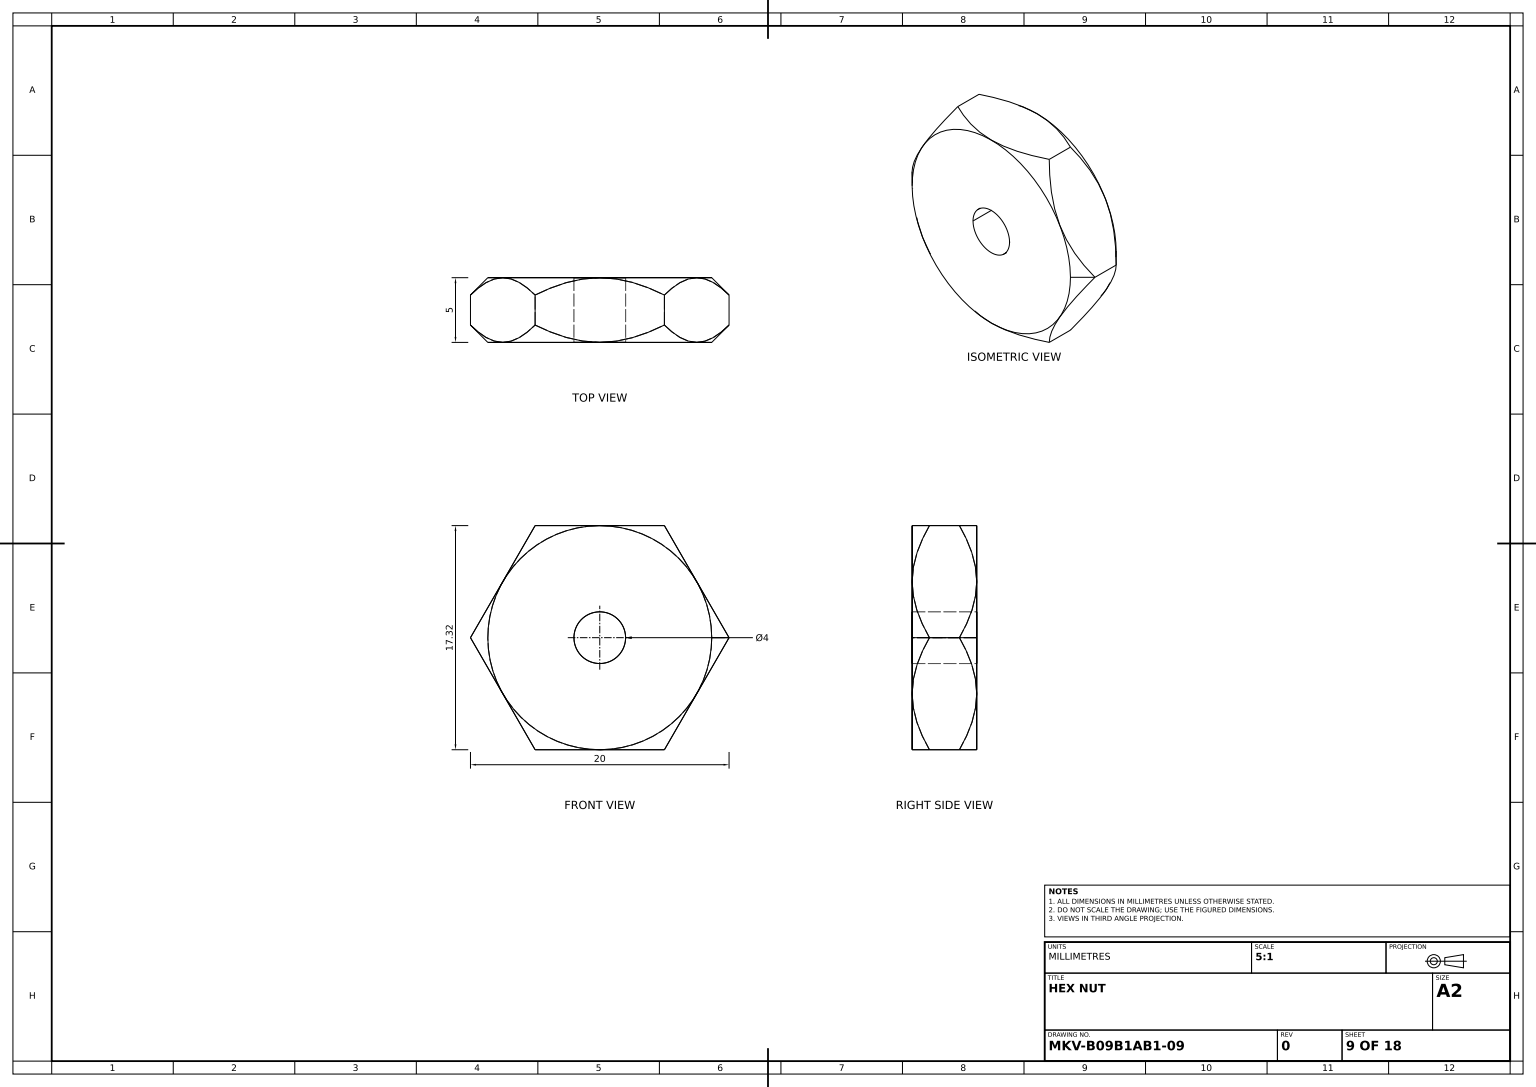
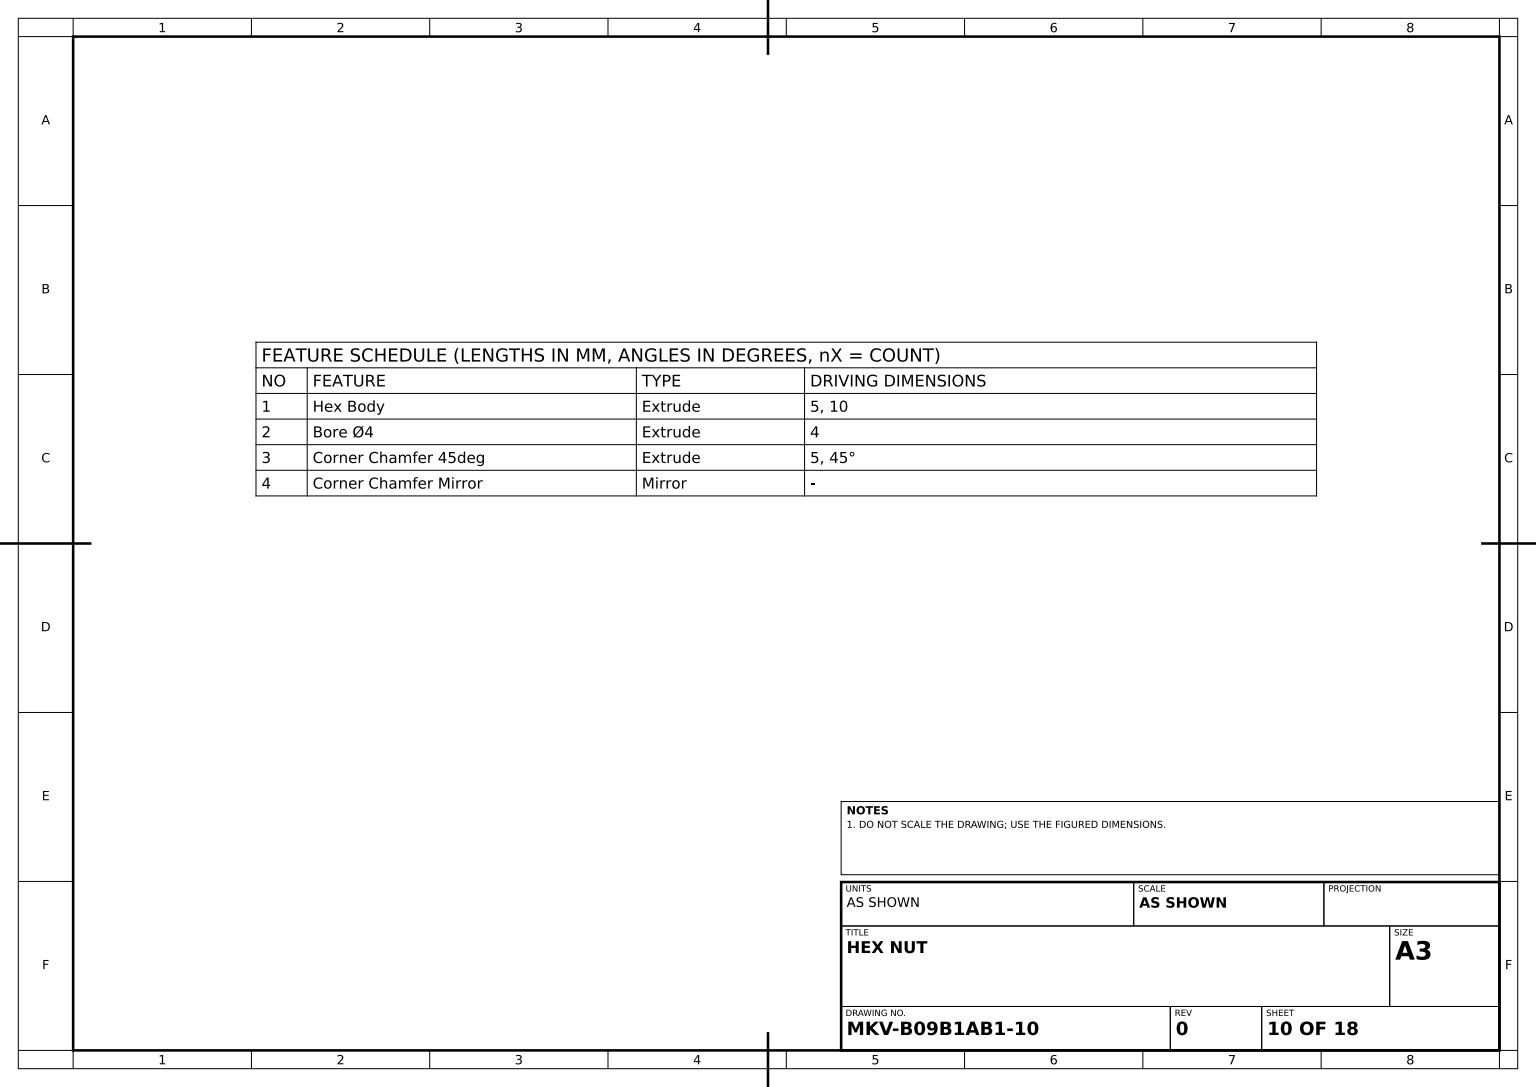
ISO-10303-21;
HEADER;
FILE_DESCRIPTION((''),'2;1');
FILE_NAME('','',(''),(''),'','','');
FILE_SCHEMA(('AUTOMOTIVE_DESIGN'));
ENDSEC;
DATA;
#1=APPLICATION_CONTEXT('');
#2=PRODUCT_CONTEXT('',#1,'mechanical');
#3=PRODUCT('','','',(#2));
#4=PRODUCT_DEFINITION_FORMATION('','',#3);
#5=PRODUCT_DEFINITION_CONTEXT('',#1,'design');
#6=PRODUCT_DEFINITION('','',#4,#5);
#7=PRODUCT_DEFINITION_SHAPE('','',#6);
#8=(LENGTH_UNIT()NAMED_UNIT(*)SI_UNIT(.MILLI.,.METRE.));
#9=(NAMED_UNIT(*)PLANE_ANGLE_UNIT()SI_UNIT($,.RADIAN.));
#10=(NAMED_UNIT(*)SI_UNIT($,.STERADIAN.)SOLID_ANGLE_UNIT());
#11=UNCERTAINTY_MEASURE_WITH_UNIT(LENGTH_MEASURE(1.E-05),#8,'distance_accuracy_value','');
#12=(GEOMETRIC_REPRESENTATION_CONTEXT(3)GLOBAL_UNCERTAINTY_ASSIGNED_CONTEXT((#11))GLOBAL_UNIT_ASSIGNED_CONTEXT((#8,#9,#10))REPRESENTATION_CONTEXT('',''));
#13=CARTESIAN_POINT('',(-5.,8.660254,1.160254));
#14=VERTEX_POINT('',#13);
#15=CARTESIAN_POINT('',(-5.,8.660254,-1.160254));
#16=VERTEX_POINT('',#15);
#17=CARTESIAN_POINT('',(-5.,8.660254,2.5));
#18=DIRECTION('',(0.,0.,-1.));
#19=VECTOR('',#18,1000.);
#20=LINE('',#17,#19);
#21=EDGE_CURVE('',#14,#16,#20,.T.);
#22=ORIENTED_EDGE('',*,*,#21,.F.);
#23=CARTESIAN_POINT('',(0.,8.660254,2.5));
#24=VERTEX_POINT('',#23);
#25=CARTESIAN_POINT('',(-0.873275,8.660254,2.5));
#26=CARTESIAN_POINT('',(-1.729188,8.660254,2.366037));
#27=CARTESIAN_POINT('',(-2.992496,8.660254,2.006453));
#28=CARTESIAN_POINT('',(-3.408399,8.660254,1.860772));
#29=CARTESIAN_POINT('',(-4.216688,8.660254,1.535097));
#30=CARTESIAN_POINT('',(-4.611749,8.660254,1.354379));
#31=B_SPLINE_CURVE_WITH_KNOTS('',3,(#23,#25,#26,#27,#28,#29,#30,#13),.UNSPECIFIED.,.F.,.F.,(4,2,2,4),(0.019209283,0.021821739,0.023127967,0.024434195),.UNSPECIFIED.);
#32=EDGE_CURVE('',#24,#14,#31,.T.);
#33=ORIENTED_EDGE('',*,*,#32,.F.);
#34=CARTESIAN_POINT('',(5.,8.660254,1.160254));
#35=VERTEX_POINT('',#34);
#36=CARTESIAN_POINT('',(4.223723,8.660254,1.548393));
#37=CARTESIAN_POINT('',(3.409694,8.660254,1.887275));
#38=CARTESIAN_POINT('',(2.159803,8.660254,2.243681));
#39=CARTESIAN_POINT('',(1.737019,8.660254,2.337768));
#40=CARTESIAN_POINT('',(0.876568,8.660254,2.466153));
#41=CARTESIAN_POINT('',(0.435084,8.660254,2.5));
#42=B_SPLINE_CURVE_WITH_KNOTS('',3,(#34,#36,#37,#38,#39,#40,#41,#23),.UNSPECIFIED.,.F.,.F.,(4,2,2,4),(0.01400296,0.016606121,0.017907702,0.019209283),.UNSPECIFIED.);
#43=EDGE_CURVE('',#35,#24,#42,.T.);
#44=ORIENTED_EDGE('',*,*,#43,.F.);
#45=CARTESIAN_POINT('',(5.,8.660254,-1.160254));
#46=VERTEX_POINT('',#45);
#47=CARTESIAN_POINT('',(5.,8.660254,2.5));
#48=LINE('',#47,#19);
#49=EDGE_CURVE('',#35,#46,#48,.T.);
#50=ORIENTED_EDGE('',*,*,#49,.T.);
#51=CARTESIAN_POINT('',(0.,8.660254,-2.5));
#52=VERTEX_POINT('',#51);
#53=CARTESIAN_POINT('',(4.223723,8.660254,-1.548393));
#54=CARTESIAN_POINT('',(3.409694,8.660254,-1.887275));
#55=CARTESIAN_POINT('',(2.159803,8.660254,-2.243681));
#56=CARTESIAN_POINT('',(1.737019,8.660254,-2.337768));
#57=CARTESIAN_POINT('',(0.876568,8.660254,-2.466153));
#58=CARTESIAN_POINT('',(0.435084,8.660254,-2.5));
#59=B_SPLINE_CURVE_WITH_KNOTS('',3,(#45,#53,#54,#55,#56,#57,#58,#51),.UNSPECIFIED.,.F.,.F.,(4,2,2,4),(0.01400296,0.016606121,0.017907702,0.019209283),.UNSPECIFIED.);
#60=EDGE_CURVE('',#46,#52,#59,.T.);
#61=ORIENTED_EDGE('',*,*,#60,.T.);
#62=CARTESIAN_POINT('',(-0.873275,8.660254,-2.5));
#63=CARTESIAN_POINT('',(-1.729188,8.660254,-2.366037));
#64=CARTESIAN_POINT('',(-2.992496,8.660254,-2.006453));
#65=CARTESIAN_POINT('',(-3.408399,8.660254,-1.860772));
#66=CARTESIAN_POINT('',(-4.216688,8.660254,-1.535097));
#67=CARTESIAN_POINT('',(-4.611749,8.660254,-1.354379));
#68=B_SPLINE_CURVE_WITH_KNOTS('',3,(#51,#62,#63,#64,#65,#66,#67,#15),.UNSPECIFIED.,.F.,.F.,(4,2,2,4),(0.019209283,0.021821739,0.023127967,0.024434195),.UNSPECIFIED.);
#69=EDGE_CURVE('',#52,#16,#68,.T.);
#70=ORIENTED_EDGE('',*,*,#69,.T.);
#71=EDGE_LOOP('',(#22,#33,#44,#50,#61,#70));
#72=FACE_OUTER_BOUND('',#71,.T.);
#73=DIRECTION('',(0.,-1.,0.));
#74=DIRECTION('',(1.,0.,0.));
#75=AXIS2_PLACEMENT_3D('',#47,#73,#74);
#76=PLANE('',#75);
#77=ADVANCED_FACE('',(#72),#76,.F.);
#78=ORIENTED_EDGE('',*,*,#69,.F.);
#79=CARTESIAN_POINT('',(-7.5,4.330127,-2.5));
#80=VERTEX_POINT('',#79);
#81=CARTESIAN_POINT('',(0.,0.,-2.5));
#82=AXIS2_PLACEMENT_3D('',#81,#18,#74);
#83=CIRCLE('',#82,8.660254);
#84=EDGE_CURVE('',#80,#52,#83,.T.);
#85=ORIENTED_EDGE('',*,*,#84,.F.);
#86=CARTESIAN_POINT('',(-5.392036,7.981228,-1.55229));
#87=CARTESIAN_POINT('',(-5.792944,7.286834,-1.885418));
#88=CARTESIAN_POINT('',(-6.415924,6.207803,-2.241594));
#89=CARTESIAN_POINT('',(-6.627224,5.841819,-2.336146));
#90=CARTESIAN_POINT('',(-7.058806,5.094297,-2.465627));
#91=CARTESIAN_POINT('',(-7.281041,4.709375,-2.5));
#92=B_SPLINE_CURVE_WITH_KNOTS('',3,(#15,#86,#87,#88,#89,#90,#91,#79),.UNSPECIFIED.,.F.,.F.,(4,2,2,4),(0.000000254,0.002591731,0.003887469,0.005183207),.UNSPECIFIED.);
#93=EDGE_CURVE('',#16,#80,#92,.T.);
#94=ORIENTED_EDGE('',*,*,#93,.F.);
#95=EDGE_LOOP('',(#78,#85,#94));
#96=FACE_OUTER_BOUND('',#95,.T.);
#97=DIRECTION('',(0.,0.,1.));
#98=AXIS2_PLACEMENT_3D('',#81,#97,#74);
#99=CONICAL_SURFACE('',#98,8.660254038,0.785398163);
#100=ADVANCED_FACE('',(#96),#99,.T.);
#101=CARTESIAN_POINT('',(-7.5,-4.330127,-2.5));
#102=VERTEX_POINT('',#101);
#103=CARTESIAN_POINT('',(-5.,-8.660254,-1.160254));
#104=VERTEX_POINT('',#103);
#105=CARTESIAN_POINT('',(-7.06515,-5.08331,-2.5));
#106=CARTESIAN_POINT('',(-6.637694,-5.823685,-2.367019));
#107=CARTESIAN_POINT('',(-5.794643,-7.283892,-1.887732));
#108=CARTESIAN_POINT('',(-5.391582,-7.982014,-1.551836));
#109=B_SPLINE_CURVE_WITH_KNOTS('',3,(#101,#105,#106,#107,#108,#103),.UNSPECIFIED.,.F.,.F.,(4,2,4),(0.005183207,0.007756532,0.010329856),.UNSPECIFIED.);
#110=EDGE_CURVE('',#102,#104,#109,.T.);
#111=ORIENTED_EDGE('',*,*,#110,.T.);
#112=CARTESIAN_POINT('',(-5.,-8.660254,1.160254));
#113=VERTEX_POINT('',#112);
#114=CARTESIAN_POINT('',(-5.,-8.660254,2.5));
#115=LINE('',#114,#19);
#116=EDGE_CURVE('',#113,#104,#115,.T.);
#117=ORIENTED_EDGE('',*,*,#116,.F.);
#118=CARTESIAN_POINT('',(-7.5,-4.330127,2.5));
#119=VERTEX_POINT('',#118);
#120=CARTESIAN_POINT('',(-7.06515,-5.08331,2.5));
#121=CARTESIAN_POINT('',(-6.637694,-5.823685,2.367019));
#122=CARTESIAN_POINT('',(-5.794643,-7.283892,1.887732));
#123=CARTESIAN_POINT('',(-5.391582,-7.982014,1.551836));
#124=B_SPLINE_CURVE_WITH_KNOTS('',3,(#118,#120,#121,#122,#123,#112),.UNSPECIFIED.,.F.,.F.,(4,2,4),(0.005183207,0.007756532,0.010329856),.UNSPECIFIED.);
#125=EDGE_CURVE('',#119,#113,#124,.T.);
#126=ORIENTED_EDGE('',*,*,#125,.F.);
#127=CARTESIAN_POINT('',(-10.,0.,1.160254));
#128=VERTEX_POINT('',#127);
#129=CARTESIAN_POINT('',(-9.607964,-0.679026,1.55229));
#130=CARTESIAN_POINT('',(-9.207056,-1.37342,1.885418));
#131=CARTESIAN_POINT('',(-8.584076,-2.452452,2.241594));
#132=CARTESIAN_POINT('',(-8.372776,-2.818435,2.336146));
#133=CARTESIAN_POINT('',(-7.941194,-3.565957,2.465627));
#134=CARTESIAN_POINT('',(-7.718959,-3.950879,2.5));
#135=B_SPLINE_CURVE_WITH_KNOTS('',3,(#127,#129,#130,#131,#132,#133,#134,#118),.UNSPECIFIED.,.F.,.F.,(4,2,2,4),(0.000000254,0.002591731,0.003887469,0.005183207),.UNSPECIFIED.);
#136=EDGE_CURVE('',#128,#119,#135,.T.);
#137=ORIENTED_EDGE('',*,*,#136,.F.);
#138=CARTESIAN_POINT('',(-10.,0.,-1.160254));
#139=VERTEX_POINT('',#138);
#140=CARTESIAN_POINT('',(-10.,0.,2.5));
#141=LINE('',#140,#19);
#142=EDGE_CURVE('',#128,#139,#141,.T.);
#143=ORIENTED_EDGE('',*,*,#142,.T.);
#144=CARTESIAN_POINT('',(-9.607964,-0.679026,-1.55229));
#145=CARTESIAN_POINT('',(-9.207056,-1.37342,-1.885418));
#146=CARTESIAN_POINT('',(-8.584076,-2.452452,-2.241594));
#147=CARTESIAN_POINT('',(-8.372776,-2.818435,-2.336146));
#148=CARTESIAN_POINT('',(-7.941194,-3.565957,-2.465627));
#149=CARTESIAN_POINT('',(-7.718959,-3.950879,-2.5));
#150=B_SPLINE_CURVE_WITH_KNOTS('',3,(#138,#144,#145,#146,#147,#148,#149,#101),.UNSPECIFIED.,.F.,.F.,(4,2,2,4),(0.000000254,0.002591731,0.003887469,0.005183207),.UNSPECIFIED.);
#151=EDGE_CURVE('',#139,#102,#150,.T.);
#152=ORIENTED_EDGE('',*,*,#151,.T.);
#153=EDGE_LOOP('',(#111,#117,#126,#137,#143,#152));
#154=FACE_OUTER_BOUND('',#153,.T.);
#155=DIRECTION('',(0.866025404,0.5,0.));
#156=DIRECTION('',(-0.5,0.866025404,0.));
#157=AXIS2_PLACEMENT_3D('',#140,#155,#156);
#158=PLANE('',#157);
#159=ADVANCED_FACE('',(#154),#158,.F.);
#160=CARTESIAN_POINT('',(-7.5,4.330127,2.5));
#161=VERTEX_POINT('',#160);
#162=CARTESIAN_POINT('',(-7.93485,3.576944,2.5));
#163=CARTESIAN_POINT('',(-8.362306,2.836569,2.367019));
#164=CARTESIAN_POINT('',(-9.205357,1.376362,1.887732));
#165=CARTESIAN_POINT('',(-9.608418,0.67824,1.551836));
#166=B_SPLINE_CURVE_WITH_KNOTS('',3,(#160,#162,#163,#164,#165,#127),.UNSPECIFIED.,.F.,.F.,(4,2,4),(0.005183207,0.007756532,0.010329856),.UNSPECIFIED.);
#167=EDGE_CURVE('',#161,#128,#166,.T.);
#168=ORIENTED_EDGE('',*,*,#167,.T.);
#169=ORIENTED_EDGE('',*,*,#136,.T.);
#170=CARTESIAN_POINT('',(0.,0.,2.5));
#171=AXIS2_PLACEMENT_3D('',#170,#97,#74);
#172=CIRCLE('',#171,8.660254);
#173=EDGE_CURVE('',#161,#119,#172,.T.);
#174=ORIENTED_EDGE('',*,*,#173,.F.);
#175=EDGE_LOOP('',(#168,#169,#174));
#176=FACE_OUTER_BOUND('',#175,.T.);
#177=AXIS2_PLACEMENT_3D('',#170,#18,#74);
#178=CONICAL_SURFACE('',#177,8.660254038,0.785398163);
#179=ADVANCED_FACE('',(#176),#178,.T.);
#180=CARTESIAN_POINT('',(7.5,-4.330127,2.5));
#181=VERTEX_POINT('',#180);
#182=CARTESIAN_POINT('',(10.,0.,1.160254));
#183=VERTEX_POINT('',#182);
#184=CARTESIAN_POINT('',(7.93485,-3.576944,2.5));
#185=CARTESIAN_POINT('',(8.362306,-2.836569,2.367019));
#186=CARTESIAN_POINT('',(9.205357,-1.376362,1.887732));
#187=CARTESIAN_POINT('',(9.608418,-0.67824,1.551836));
#188=B_SPLINE_CURVE_WITH_KNOTS('',3,(#180,#184,#185,#186,#187,#182),.UNSPECIFIED.,.F.,.F.,(4,2,4),(0.005183207,0.007756532,0.010329856),.UNSPECIFIED.);
#189=EDGE_CURVE('',#181,#183,#188,.T.);
#190=ORIENTED_EDGE('',*,*,#189,.T.);
#191=CARTESIAN_POINT('',(8.660254,0.,2.5));
#192=VERTEX_POINT('',#191);
#193=DIRECTION('',(0.707106781,0.,-0.707106781));
#194=VECTOR('',#193,1000.);
#195=LINE('',#191,#194);
#196=EDGE_CURVE('',#192,#183,#195,.T.);
#197=ORIENTED_EDGE('',*,*,#196,.F.);
#198=EDGE_CURVE('',#181,#192,#172,.T.);
#199=ORIENTED_EDGE('',*,*,#198,.F.);
#200=EDGE_LOOP('',(#190,#197,#199));
#201=FACE_OUTER_BOUND('',#200,.T.);
#202=ADVANCED_FACE('',(#201),#178,.T.);
#203=ORIENTED_EDGE('',*,*,#125,.T.);
#204=CARTESIAN_POINT('',(0.,-8.660254,2.5));
#205=VERTEX_POINT('',#204);
#206=CARTESIAN_POINT('',(-4.223723,-8.660254,1.548393));
#207=CARTESIAN_POINT('',(-3.409694,-8.660254,1.887275));
#208=CARTESIAN_POINT('',(-2.159803,-8.660254,2.243681));
#209=CARTESIAN_POINT('',(-1.737019,-8.660254,2.337768));
#210=CARTESIAN_POINT('',(-0.876568,-8.660254,2.466153));
#211=CARTESIAN_POINT('',(-0.435084,-8.660254,2.5));
#212=B_SPLINE_CURVE_WITH_KNOTS('',3,(#112,#206,#207,#208,#209,#210,#211,#204),.UNSPECIFIED.,.F.,.F.,(4,2,2,4),(0.01400296,0.016606121,0.017907702,0.019209283),.UNSPECIFIED.);
#213=EDGE_CURVE('',#113,#205,#212,.T.);
#214=ORIENTED_EDGE('',*,*,#213,.T.);
#215=EDGE_CURVE('',#119,#205,#172,.T.);
#216=ORIENTED_EDGE('',*,*,#215,.F.);
#217=EDGE_LOOP('',(#203,#214,#216));
#218=FACE_OUTER_BOUND('',#217,.T.);
#219=ADVANCED_FACE('',(#218),#178,.T.);
#220=ORIENTED_EDGE('',*,*,#116,.T.);
#221=CARTESIAN_POINT('',(0.,-8.660254,-2.5));
#222=VERTEX_POINT('',#221);
#223=CARTESIAN_POINT('',(-4.223723,-8.660254,-1.548393));
#224=CARTESIAN_POINT('',(-3.409694,-8.660254,-1.887275));
#225=CARTESIAN_POINT('',(-2.159803,-8.660254,-2.243681));
#226=CARTESIAN_POINT('',(-1.737019,-8.660254,-2.337768));
#227=CARTESIAN_POINT('',(-0.876568,-8.660254,-2.466153));
#228=CARTESIAN_POINT('',(-0.435084,-8.660254,-2.5));
#229=B_SPLINE_CURVE_WITH_KNOTS('',3,(#103,#223,#224,#225,#226,#227,#228,#221),.UNSPECIFIED.,.F.,.F.,(4,2,2,4),(0.01400296,0.016606121,0.017907702,0.019209283),.UNSPECIFIED.);
#230=EDGE_CURVE('',#104,#222,#229,.T.);
#231=ORIENTED_EDGE('',*,*,#230,.T.);
#232=CARTESIAN_POINT('',(5.,-8.660254,-1.160254));
#233=VERTEX_POINT('',#232);
#234=CARTESIAN_POINT('',(0.873275,-8.660254,-2.5));
#235=CARTESIAN_POINT('',(1.729188,-8.660254,-2.366037));
#236=CARTESIAN_POINT('',(2.992496,-8.660254,-2.006453));
#237=CARTESIAN_POINT('',(3.408399,-8.660254,-1.860772));
#238=CARTESIAN_POINT('',(4.216688,-8.660254,-1.535097));
#239=CARTESIAN_POINT('',(4.611749,-8.660254,-1.354379));
#240=B_SPLINE_CURVE_WITH_KNOTS('',3,(#221,#234,#235,#236,#237,#238,#239,#232),.UNSPECIFIED.,.F.,.F.,(4,2,2,4),(0.019209283,0.021821739,0.023127967,0.024434195),.UNSPECIFIED.);
#241=EDGE_CURVE('',#222,#233,#240,.T.);
#242=ORIENTED_EDGE('',*,*,#241,.T.);
#243=CARTESIAN_POINT('',(5.,-8.660254,1.160254));
#244=VERTEX_POINT('',#243);
#245=CARTESIAN_POINT('',(5.,-8.660254,2.5));
#246=LINE('',#245,#19);
#247=EDGE_CURVE('',#244,#233,#246,.T.);
#248=ORIENTED_EDGE('',*,*,#247,.F.);
#249=CARTESIAN_POINT('',(0.873275,-8.660254,2.5));
#250=CARTESIAN_POINT('',(1.729188,-8.660254,2.366037));
#251=CARTESIAN_POINT('',(2.992496,-8.660254,2.006453));
#252=CARTESIAN_POINT('',(3.408399,-8.660254,1.860772));
#253=CARTESIAN_POINT('',(4.216688,-8.660254,1.535097));
#254=CARTESIAN_POINT('',(4.611749,-8.660254,1.354379));
#255=B_SPLINE_CURVE_WITH_KNOTS('',3,(#204,#249,#250,#251,#252,#253,#254,#243),.UNSPECIFIED.,.F.,.F.,(4,2,2,4),(0.019209283,0.021821739,0.023127967,0.024434195),.UNSPECIFIED.);
#256=EDGE_CURVE('',#205,#244,#255,.T.);
#257=ORIENTED_EDGE('',*,*,#256,.F.);
#258=ORIENTED_EDGE('',*,*,#213,.F.);
#259=EDGE_LOOP('',(#220,#231,#242,#248,#257,#258));
#260=FACE_OUTER_BOUND('',#259,.T.);
#261=DIRECTION('',(0.,1.,0.));
#262=DIRECTION('',(-1.,0.,0.));
#263=AXIS2_PLACEMENT_3D('',#114,#261,#262);
#264=PLANE('',#263);
#265=ADVANCED_FACE('',(#260),#264,.F.);
#266=CARTESIAN_POINT('',(2.,0.,-2.5));
#267=VERTEX_POINT('',#266);
#268=CARTESIAN_POINT('',(-2.,0.,-2.5));
#269=VERTEX_POINT('',#268);
#270=CIRCLE('',#98,2.);
#271=EDGE_CURVE('',#267,#269,#270,.T.);
#272=ORIENTED_EDGE('',*,*,#271,.F.);
#273=CARTESIAN_POINT('',(2.,0.,2.5));
#274=VERTEX_POINT('',#273);
#275=VECTOR('',#97,1000.);
#276=LINE('',#266,#275);
#277=EDGE_CURVE('',#267,#274,#276,.T.);
#278=ORIENTED_EDGE('',*,*,#277,.T.);
#279=CARTESIAN_POINT('',(-2.,0.,2.5));
#280=VERTEX_POINT('',#279);
#281=CIRCLE('',#171,2.);
#282=EDGE_CURVE('',#274,#280,#281,.T.);
#283=ORIENTED_EDGE('',*,*,#282,.T.);
#284=LINE('',#268,#275);
#285=EDGE_CURVE('',#269,#280,#284,.T.);
#286=ORIENTED_EDGE('',*,*,#285,.F.);
#287=EDGE_LOOP('',(#272,#278,#283,#286));
#288=FACE_OUTER_BOUND('',#287,.T.);
#289=CYLINDRICAL_SURFACE('',#98,2.);
#290=ADVANCED_FACE('',(#288),#289,.F.);
#291=EDGE_CURVE('',#269,#267,#270,.T.);
#292=ORIENTED_EDGE('',*,*,#291,.T.);
#293=ORIENTED_EDGE('',*,*,#271,.T.);
#294=EDGE_LOOP('',(#292,#293));
#295=FACE_BOUND('',#294,.T.);
#296=CARTESIAN_POINT('',(7.5,4.330127,-2.5));
#297=VERTEX_POINT('',#296);
#298=CIRCLE('',#98,8.660254);
#299=EDGE_CURVE('',#297,#52,#298,.T.);
#300=ORIENTED_EDGE('',*,*,#299,.F.);
#301=CARTESIAN_POINT('',(8.660254,0.,-2.5));
#302=VERTEX_POINT('',#301);
#303=EDGE_CURVE('',#297,#302,#83,.T.);
#304=ORIENTED_EDGE('',*,*,#303,.T.);
#305=CARTESIAN_POINT('',(7.5,-4.330127,-2.5));
#306=VERTEX_POINT('',#305);
#307=EDGE_CURVE('',#302,#306,#83,.T.);
#308=ORIENTED_EDGE('',*,*,#307,.T.);
#309=EDGE_CURVE('',#306,#222,#83,.T.);
#310=ORIENTED_EDGE('',*,*,#309,.T.);
#311=EDGE_CURVE('',#222,#102,#83,.T.);
#312=ORIENTED_EDGE('',*,*,#311,.T.);
#313=EDGE_CURVE('',#102,#80,#83,.T.);
#314=ORIENTED_EDGE('',*,*,#313,.T.);
#315=ORIENTED_EDGE('',*,*,#84,.T.);
#316=EDGE_LOOP('',(#300,#304,#308,#310,#312,#314,#315));
#317=FACE_OUTER_BOUND('',#316,.T.);
#318=PLANE('',#98);
#319=ADVANCED_FACE('',(#295,#317),#318,.F.);
#320=CARTESIAN_POINT('',(10.,0.,-1.160254));
#321=VERTEX_POINT('',#320);
#322=CARTESIAN_POINT('',(10.,0.,2.5));
#323=LINE('',#322,#19);
#324=EDGE_CURVE('',#183,#321,#323,.T.);
#325=ORIENTED_EDGE('',*,*,#324,.T.);
#326=CARTESIAN_POINT('',(9.607964,0.679026,-1.55229));
#327=CARTESIAN_POINT('',(9.207056,1.37342,-1.885418));
#328=CARTESIAN_POINT('',(8.584076,2.452452,-2.241594));
#329=CARTESIAN_POINT('',(8.372776,2.818435,-2.336146));
#330=CARTESIAN_POINT('',(7.941194,3.565957,-2.465627));
#331=CARTESIAN_POINT('',(7.718959,3.950879,-2.5));
#332=B_SPLINE_CURVE_WITH_KNOTS('',3,(#320,#326,#327,#328,#329,#330,#331,#296),.UNSPECIFIED.,.F.,.F.,(4,2,2,4),(0.000000254,0.002591731,0.003887469,0.005183207),.UNSPECIFIED.);
#333=EDGE_CURVE('',#321,#297,#332,.T.);
#334=ORIENTED_EDGE('',*,*,#333,.T.);
#335=CARTESIAN_POINT('',(7.06515,5.08331,-2.5));
#336=CARTESIAN_POINT('',(6.637694,5.823685,-2.367019));
#337=CARTESIAN_POINT('',(5.794643,7.283892,-1.887732));
#338=CARTESIAN_POINT('',(5.391582,7.982014,-1.551836));
#339=B_SPLINE_CURVE_WITH_KNOTS('',3,(#296,#335,#336,#337,#338,#45),.UNSPECIFIED.,.F.,.F.,(4,2,4),(0.005183207,0.007756532,0.010329856),.UNSPECIFIED.);
#340=EDGE_CURVE('',#297,#46,#339,.T.);
#341=ORIENTED_EDGE('',*,*,#340,.T.);
#342=ORIENTED_EDGE('',*,*,#49,.F.);
#343=CARTESIAN_POINT('',(7.5,4.330127,2.5));
#344=VERTEX_POINT('',#343);
#345=CARTESIAN_POINT('',(7.06515,5.08331,2.5));
#346=CARTESIAN_POINT('',(6.637694,5.823685,2.367019));
#347=CARTESIAN_POINT('',(5.794643,7.283892,1.887732));
#348=CARTESIAN_POINT('',(5.391582,7.982014,1.551836));
#349=B_SPLINE_CURVE_WITH_KNOTS('',3,(#343,#345,#346,#347,#348,#34),.UNSPECIFIED.,.F.,.F.,(4,2,4),(0.005183207,0.007756532,0.010329856),.UNSPECIFIED.);
#350=EDGE_CURVE('',#344,#35,#349,.T.);
#351=ORIENTED_EDGE('',*,*,#350,.F.);
#352=CARTESIAN_POINT('',(9.607964,0.679026,1.55229));
#353=CARTESIAN_POINT('',(9.207056,1.37342,1.885418));
#354=CARTESIAN_POINT('',(8.584076,2.452452,2.241594));
#355=CARTESIAN_POINT('',(8.372776,2.818435,2.336146));
#356=CARTESIAN_POINT('',(7.941194,3.565957,2.465627));
#357=CARTESIAN_POINT('',(7.718959,3.950879,2.5));
#358=B_SPLINE_CURVE_WITH_KNOTS('',3,(#182,#352,#353,#354,#355,#356,#357,#343),.UNSPECIFIED.,.F.,.F.,(4,2,2,4),(0.000000254,0.002591731,0.003887469,0.005183207),.UNSPECIFIED.);
#359=EDGE_CURVE('',#183,#344,#358,.T.);
#360=ORIENTED_EDGE('',*,*,#359,.F.);
#361=EDGE_LOOP('',(#325,#334,#341,#342,#351,#360));
#362=FACE_OUTER_BOUND('',#361,.T.);
#363=DIRECTION('',(-0.866025404,-0.5,0.));
#364=DIRECTION('',(0.5,-0.866025404,0.));
#365=AXIS2_PLACEMENT_3D('',#322,#363,#364);
#366=PLANE('',#365);
#367=ADVANCED_FACE('',(#362),#366,.F.);
#368=ORIENTED_EDGE('',*,*,#333,.F.);
#369=DIRECTION('',(0.707106781,0.,0.707106781));
#370=VECTOR('',#369,1000.);
#371=LINE('',#301,#370);
#372=EDGE_CURVE('',#302,#321,#371,.T.);
#373=ORIENTED_EDGE('',*,*,#372,.F.);
#374=ORIENTED_EDGE('',*,*,#303,.F.);
#375=EDGE_LOOP('',(#368,#373,#374));
#376=FACE_OUTER_BOUND('',#375,.T.);
#377=ADVANCED_FACE('',(#376),#99,.T.);
#378=EDGE_CURVE('',#192,#344,#172,.T.);
#379=ORIENTED_EDGE('',*,*,#378,.F.);
#380=ORIENTED_EDGE('',*,*,#196,.T.);
#381=ORIENTED_EDGE('',*,*,#359,.T.);
#382=EDGE_LOOP('',(#379,#380,#381));
#383=FACE_OUTER_BOUND('',#382,.T.);
#384=ADVANCED_FACE('',(#383),#178,.T.);
#385=ORIENTED_EDGE('',*,*,#311,.F.);
#386=ORIENTED_EDGE('',*,*,#230,.F.);
#387=ORIENTED_EDGE('',*,*,#110,.F.);
#388=EDGE_LOOP('',(#385,#386,#387));
#389=FACE_OUTER_BOUND('',#388,.T.);
#390=ADVANCED_FACE('',(#389),#99,.T.);
#391=ORIENTED_EDGE('',*,*,#340,.F.);
#392=ORIENTED_EDGE('',*,*,#299,.T.);
#393=ORIENTED_EDGE('',*,*,#60,.F.);
#394=EDGE_LOOP('',(#391,#392,#393));
#395=FACE_OUTER_BOUND('',#394,.T.);
#396=ADVANCED_FACE('',(#395),#99,.T.);
#397=ORIENTED_EDGE('',*,*,#93,.T.);
#398=CARTESIAN_POINT('',(-7.93485,3.576944,-2.5));
#399=CARTESIAN_POINT('',(-8.362306,2.836569,-2.367019));
#400=CARTESIAN_POINT('',(-9.205357,1.376362,-1.887732));
#401=CARTESIAN_POINT('',(-9.608418,0.67824,-1.551836));
#402=B_SPLINE_CURVE_WITH_KNOTS('',3,(#79,#398,#399,#400,#401,#138),.UNSPECIFIED.,.F.,.F.,(4,2,4),(0.005183207,0.007756532,0.010329856),.UNSPECIFIED.);
#403=EDGE_CURVE('',#80,#139,#402,.T.);
#404=ORIENTED_EDGE('',*,*,#403,.T.);
#405=ORIENTED_EDGE('',*,*,#142,.F.);
#406=ORIENTED_EDGE('',*,*,#167,.F.);
#407=CARTESIAN_POINT('',(-5.392036,7.981228,1.55229));
#408=CARTESIAN_POINT('',(-5.792944,7.286834,1.885418));
#409=CARTESIAN_POINT('',(-6.415924,6.207803,2.241594));
#410=CARTESIAN_POINT('',(-6.627224,5.841819,2.336146));
#411=CARTESIAN_POINT('',(-7.058806,5.094297,2.465627));
#412=CARTESIAN_POINT('',(-7.281041,4.709375,2.5));
#413=B_SPLINE_CURVE_WITH_KNOTS('',3,(#13,#407,#408,#409,#410,#411,#412,#160),.UNSPECIFIED.,.F.,.F.,(4,2,2,4),(0.000000254,0.002591731,0.003887469,0.005183207),.UNSPECIFIED.);
#414=EDGE_CURVE('',#14,#161,#413,.T.);
#415=ORIENTED_EDGE('',*,*,#414,.F.);
#416=ORIENTED_EDGE('',*,*,#21,.T.);
#417=EDGE_LOOP('',(#397,#404,#405,#406,#415,#416));
#418=FACE_OUTER_BOUND('',#417,.T.);
#419=DIRECTION('',(0.866025404,-0.5,0.));
#420=DIRECTION('',(0.5,0.866025404,0.));
#421=AXIS2_PLACEMENT_3D('',#17,#419,#420);
#422=PLANE('',#421);
#423=ADVANCED_FACE('',(#418),#422,.F.);
#424=ORIENTED_EDGE('',*,*,#247,.T.);
#425=CARTESIAN_POINT('',(5.392036,-7.981228,-1.55229));
#426=CARTESIAN_POINT('',(5.792944,-7.286834,-1.885418));
#427=CARTESIAN_POINT('',(6.415924,-6.207803,-2.241594));
#428=CARTESIAN_POINT('',(6.627224,-5.841819,-2.336146));
#429=CARTESIAN_POINT('',(7.058806,-5.094297,-2.465627));
#430=CARTESIAN_POINT('',(7.281041,-4.709375,-2.5));
#431=B_SPLINE_CURVE_WITH_KNOTS('',3,(#232,#425,#426,#427,#428,#429,#430,#305),.UNSPECIFIED.,.F.,.F.,(4,2,2,4),(0.000000254,0.002591731,0.003887469,0.005183207),.UNSPECIFIED.);
#432=EDGE_CURVE('',#233,#306,#431,.T.);
#433=ORIENTED_EDGE('',*,*,#432,.T.);
#434=CARTESIAN_POINT('',(7.93485,-3.576944,-2.5));
#435=CARTESIAN_POINT('',(8.362306,-2.836569,-2.367019));
#436=CARTESIAN_POINT('',(9.205357,-1.376362,-1.887732));
#437=CARTESIAN_POINT('',(9.608418,-0.67824,-1.551836));
#438=B_SPLINE_CURVE_WITH_KNOTS('',3,(#305,#434,#435,#436,#437,#320),.UNSPECIFIED.,.F.,.F.,(4,2,4),(0.005183207,0.007756532,0.010329856),.UNSPECIFIED.);
#439=EDGE_CURVE('',#306,#321,#438,.T.);
#440=ORIENTED_EDGE('',*,*,#439,.T.);
#441=ORIENTED_EDGE('',*,*,#324,.F.);
#442=ORIENTED_EDGE('',*,*,#189,.F.);
#443=CARTESIAN_POINT('',(5.392036,-7.981228,1.55229));
#444=CARTESIAN_POINT('',(5.792944,-7.286834,1.885418));
#445=CARTESIAN_POINT('',(6.415924,-6.207803,2.241594));
#446=CARTESIAN_POINT('',(6.627224,-5.841819,2.336146));
#447=CARTESIAN_POINT('',(7.058806,-5.094297,2.465627));
#448=CARTESIAN_POINT('',(7.281041,-4.709375,2.5));
#449=B_SPLINE_CURVE_WITH_KNOTS('',3,(#243,#443,#444,#445,#446,#447,#448,#180),.UNSPECIFIED.,.F.,.F.,(4,2,2,4),(0.000000254,0.002591731,0.003887469,0.005183207),.UNSPECIFIED.);
#450=EDGE_CURVE('',#244,#181,#449,.T.);
#451=ORIENTED_EDGE('',*,*,#450,.F.);
#452=EDGE_LOOP('',(#424,#433,#440,#441,#442,#451));
#453=FACE_OUTER_BOUND('',#452,.T.);
#454=DIRECTION('',(-0.866025404,0.5,0.));
#455=DIRECTION('',(-0.5,-0.866025404,0.));
#456=AXIS2_PLACEMENT_3D('',#245,#454,#455);
#457=PLANE('',#456);
#458=ADVANCED_FACE('',(#453),#457,.F.);
#459=ORIENTED_EDGE('',*,*,#350,.T.);
#460=ORIENTED_EDGE('',*,*,#43,.T.);
#461=EDGE_CURVE('',#344,#24,#172,.T.);
#462=ORIENTED_EDGE('',*,*,#461,.F.);
#463=EDGE_LOOP('',(#459,#460,#462));
#464=FACE_OUTER_BOUND('',#463,.T.);
#465=ADVANCED_FACE('',(#464),#178,.T.);
#466=ORIENTED_EDGE('',*,*,#282,.F.);
#467=EDGE_CURVE('',#280,#274,#281,.T.);
#468=ORIENTED_EDGE('',*,*,#467,.F.);
#469=EDGE_LOOP('',(#466,#468));
#470=FACE_BOUND('',#469,.T.);
#471=ORIENTED_EDGE('',*,*,#173,.T.);
#472=ORIENTED_EDGE('',*,*,#215,.T.);
#473=EDGE_CURVE('',#205,#181,#172,.T.);
#474=ORIENTED_EDGE('',*,*,#473,.T.);
#475=ORIENTED_EDGE('',*,*,#198,.T.);
#476=ORIENTED_EDGE('',*,*,#378,.T.);
#477=ORIENTED_EDGE('',*,*,#461,.T.);
#478=EDGE_CURVE('',#24,#161,#172,.T.);
#479=ORIENTED_EDGE('',*,*,#478,.T.);
#480=EDGE_LOOP('',(#471,#472,#474,#475,#476,#477,#479));
#481=FACE_OUTER_BOUND('',#480,.T.);
#482=PLANE('',#171);
#483=ADVANCED_FACE('',(#470,#481),#482,.T.);
#484=ORIENTED_EDGE('',*,*,#403,.F.);
#485=ORIENTED_EDGE('',*,*,#313,.F.);
#486=ORIENTED_EDGE('',*,*,#151,.F.);
#487=EDGE_LOOP('',(#484,#485,#486));
#488=FACE_OUTER_BOUND('',#487,.T.);
#489=ADVANCED_FACE('',(#488),#99,.T.);
#490=ORIENTED_EDGE('',*,*,#467,.T.);
#491=ORIENTED_EDGE('',*,*,#277,.F.);
#492=ORIENTED_EDGE('',*,*,#291,.F.);
#493=ORIENTED_EDGE('',*,*,#285,.T.);
#494=EDGE_LOOP('',(#490,#491,#492,#493));
#495=FACE_OUTER_BOUND('',#494,.T.);
#496=ADVANCED_FACE('',(#495),#289,.F.);
#497=ORIENTED_EDGE('',*,*,#414,.T.);
#498=ORIENTED_EDGE('',*,*,#478,.F.);
#499=ORIENTED_EDGE('',*,*,#32,.T.);
#500=EDGE_LOOP('',(#497,#498,#499));
#501=FACE_OUTER_BOUND('',#500,.T.);
#502=ADVANCED_FACE('',(#501),#178,.T.);
#503=ORIENTED_EDGE('',*,*,#372,.T.);
#504=ORIENTED_EDGE('',*,*,#439,.F.);
#505=ORIENTED_EDGE('',*,*,#307,.F.);
#506=EDGE_LOOP('',(#503,#504,#505));
#507=FACE_OUTER_BOUND('',#506,.T.);
#508=ADVANCED_FACE('',(#507),#99,.T.);
#509=ORIENTED_EDGE('',*,*,#256,.T.);
#510=ORIENTED_EDGE('',*,*,#450,.T.);
#511=ORIENTED_EDGE('',*,*,#473,.F.);
#512=EDGE_LOOP('',(#509,#510,#511));
#513=FACE_OUTER_BOUND('',#512,.T.);
#514=ADVANCED_FACE('',(#513),#178,.T.);
#515=ORIENTED_EDGE('',*,*,#241,.F.);
#516=ORIENTED_EDGE('',*,*,#309,.F.);
#517=ORIENTED_EDGE('',*,*,#432,.F.);
#518=EDGE_LOOP('',(#515,#516,#517));
#519=FACE_OUTER_BOUND('',#518,.T.);
#520=ADVANCED_FACE('',(#519),#99,.T.);
#521=CLOSED_SHELL('',(#77,#100,#159,#179,#202,#219,#265,#290,#319,#367,#377,#384,#390,#396,#423,#458,#465,#483,#489,#496,#502,#508,#514,#520));
#522=MANIFOLD_SOLID_BREP('',#521);
#523=ADVANCED_BREP_SHAPE_REPRESENTATION('',(#522),#12);
#524=SHAPE_DEFINITION_REPRESENTATION(#7,#523);
ENDSEC;
END-ISO-10303-21;
